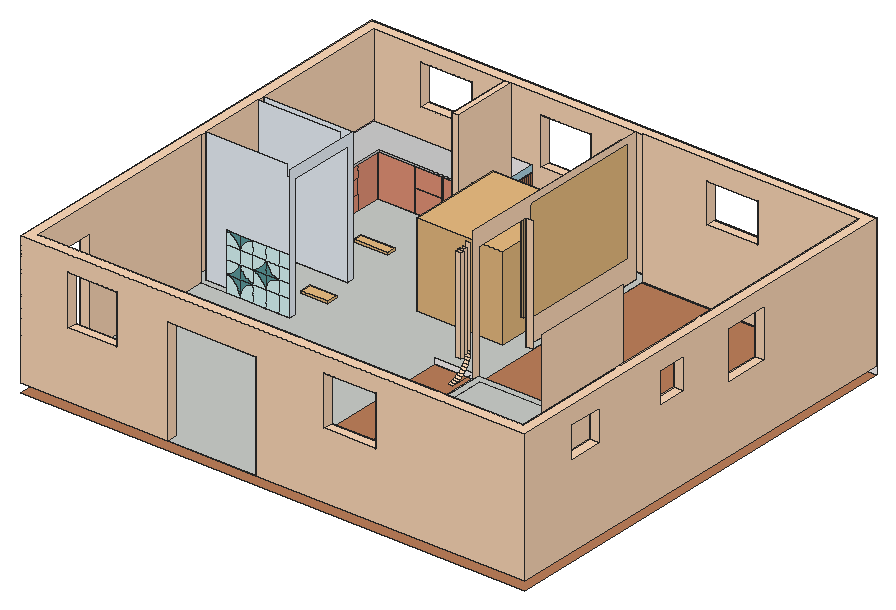
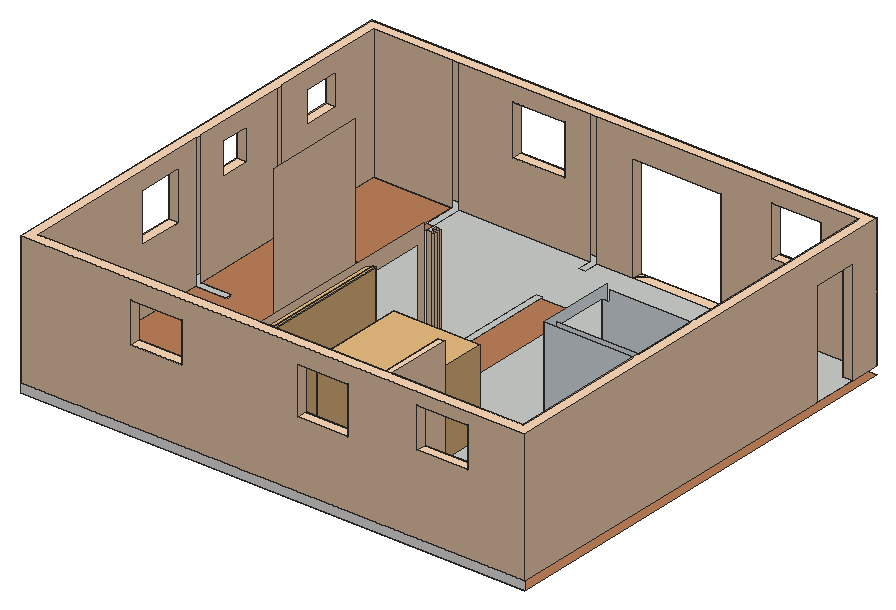
# SketchUp Ruby script. Lengths in inches.
U = 1.inch
M = Sketchup.active_model
def pt(a) = Geom::Point3d.new(a.map { |v| v * U })
def face(e, loops, mat)
  f = e.add_face(loops[0].map { |a| pt(a) })
  loops[1..].each { |l| e.add_face(l.map { |a| pt(a) }).erase! }
  f.material = f.back_material = mat if mat
  f
end
# faces: each face lists its corners as indices into pts; further lists are holes
def faces(e, pts, list, mat = nil) = list.each { |f| face(e, (f[0].is_a?(Array) ? f : [f]).map { |l| l.map { |i| pts[i] } }, mat) }
# xy, xz, yz: faces in a plane at the given z, y or x. An outline is a flat list of corners, or four numbers for a rectangle; further outlines are holes
def ring(l) = l.size == 4 ? [[l[0], l[1]], [l[2], l[1]], [l[2], l[3]], [l[0], l[3]]] : l.each_slice(2).to_a
def flat(e, list, mat, &to3) = list.each { |f| face(e, (f[0].is_a?(Array) ? f : [f]).map { |l| ring(l).map { |u, v| to3.(u, v) } }, mat) }
def xy(e, z, list, mat = nil) = flat(e, list, mat) { |x, y| [x, y, z] }
def xz(e, y, list, mat = nil) = flat(e, list, mat) { |x, z| [x, y, z] }
def yz(e, x, list, mat = nil) = flat(e, list, mat) { |y, z| [x, y, z] }
def lines(e, pts, list) = list.each { |a, b| e.add_line(pt(pts[a]), pt(pts[b])) }
# prism: a flat outline (further loops are holes) pulled along v
def prism(e, loops, v, mat = nil)
  f = face(e, loops, mat); d = Geom::Vector3d.new(v.map { |x| x * U })
  f.pushpull(f.normal.samedirection?(d) ? d.length : -d.length)
end
def box(e, o, s, mat = nil) = prism(e, [[o, [o[0] + s[0], o[1], o[2]], [o[0] + s[0], o[1] + s[1], o[2]], [o[0], o[1] + s[1], o[2]]]], [0, 0, s[2]], mat)
def at(x, y, z, deg = 0) = Geom::Transformation.translation(pt([x, y, z])) * Geom::Transformation.rotation(ORIGIN, Z_AXIS, deg.degrees)
def axes(o, x, y, z) = Geom::Transformation.new([*x, 0, *y, 0, *z, 0, *pt(o).to_a, 1])
def part(name) = M.definitions.add(name)
# library, detail: a bought-in or finely detailed component or shape, given as its bounding box
def library(name, o, s) = part(name).tap { |d| box(d.entities, o, s) }
def detail(e, o, s) = box(e.add_group.entities, o, s)
def put(e, d, t, mat = nil) = e.add_instance(d, t).tap { |i| i.material = mat if mat }
def group(e, t, mat = nil) = e.add_group.tap { |g| g.transformation = t; g.material = mat if mat }.entities
root = M.entities
M.materials.add("3D66_SU_1584934530570_001").color = [198, 166, 120]
M.materials.add("[0006_Pink]").color = [255, 192, 203]
M.materials.add("[0010_Snow]").color = [255, 250, 250]
M.materials.add("[0014_DarkSalmon]").color = [233, 150, 122]
M.materials.add("[0027_PeachPuff]").color = [255, 218, 185]
M.materials.add("[0081_CadetBlue]").color = [95, 158, 160]
M.materials.add("[0090_LightCyan]").color = [224, 255, 255]
M.materials.add("[0093_AliceBlue]").color = [240, 248, 255]
M.materials.add("[0095_LightBlue]").color = [173, 216, 230]
M.materials.add("[Basic Tile]").color = [203, 206, 202]
M.materials.add("[Carrera Marble]").color = [207, 207, 207]
M.materials.add("[Wood Veneer 02]").color = [190, 128, 91]
c1 = library("kitchen",[0.875,0,0],[30.86,8.22,2])
c2 = library("pooja",[0.875,0,0],[24.44,10.22,2])
c3 = library("Dining table set",[0,0,0],[63.25,59.01,43.49])
c4 = library("Dining ar",[0.98,0,0],[40.63,10.22,2])
c5 = part("\#79\#1")
prism(c5.entities,[[[1108.05,3703.68,-100.79],[497.03,3703.68,-100.79],[497.03,5166.16,-100.79],[1108.05,5166.16,-100.79]],[[1097.77,5155.88,-100.79],[507.31,5155.88,-100.79],[507.31,3713.96,-100.79],[1097.77,3713.96,-100.79]]],[0,0,14.57],"3D66_SU_1584934530570_001")
c6 = library("\#81",[507.31,3713.96,-116.94],[590.46,1441.92,47.04])
xy(root,-7.5625,[[109.5625,138.9375,571.5625,540.9375]],"[Wood Veneer 02]")
xy(root,0,[[[109.5625,138.9375,571.5625,540.9375],[490.5625,258.9375,490.5625,347.21,492.04,347.21,492.04,350.1875,490.5625,350.1875,490.5625,351.9375,364.5625,351.9375,364.5625,531.9375,562.5625,531.9375,562.5625,351.9375,534.83,351.9375,534.83,350.1875,533.35,350.1875,533.35,348.7,535.05,348.7,535.05,345.9375,562.5625,345.9375,562.5625,258.9375],[490.5625,147.9375,490.5625,177.19,483.52,177.19,483.52,240.51,490.5625,240.51,490.5625,252.9375,562.5625,252.9375,562.5625,147.9375],[323.75,211.625,358.5625,345.9375],[118.5625,405.9375,139.41,531.9375],[244.5625,486.17,263.2,531.9375]]],"[Basic Tile]")
xy(root,6.75,[[263.2,488.05,263.89,509.17],[263.89,488.05,264.76,489.21],[263.89,490.54,264.76,491.71],[263.89,493.04,264.76,494.2],[263.89,495.53,264.76,496.7],
  [263.89,498.03,264.76,499.19],[263.89,500.52,264.76,501.6875],[263.89,503.02,264.76,504.18],[263.89,505.51,264.76,506.68],[263.89,508.01,264.76,509.17],
  [263.2,509.67,263.89,530],[263.89,510.01,264.76,511.17],[263.89,512.36,264.76,513.53],[263.89,514.71,264.76,515.88],[263.89,517.07,264.76,518.23],
  [263.89,519.42,264.76,520.59],[263.89,521.77,264.76,522.9375],[263.89,524.125,264.76,525.29],[263.89,526.48,264.76,527.65],[263.89,528.83,264.76,530]],"[0010_Snow]")
xy(root,23.08,[[354.3125,330.97,359.375,333.97],[354.3125,336.47,357.4375,339.47]],"[0027_PeachPuff]")
xy(root,44.75,[[118.58,405.9375,118.58,533.96,238.5625,533.96,238.5625,500.54,148.4,500.54,148.4,405.9375]],"[0006_Pink]")
xy(root,46.25,[[118.58,405.9375,148.4,405.9375,148.4,500.54,238.5625,500.54,238.5625,533.96,118.58,533.96]],"[Carrera Marble]")
xy(root,121.1875,[[238.5625,471.5,244.5625,531.9375]],"[0027_PeachPuff]")
xz(root,330.97,[[354.3125,23.08,359.375,110.27]],"[0027_PeachPuff]")
xz(root,333.9375,[[154.5625,0,154.5625,15.41,142.5625,15.41,144.1875,14.8125,145.74,14.05,147.22,13.14,148.59,12.09,149.85,10.9,150.98,9.59,151.97,8.17,152.82,6.66,153.5,5.07,154.03,3.42,154.38,1.72],[154.5625,0,154.6875,1.74,155,3.46,155.49,5.13,156.16,6.74,157,8.27,158,9.7,159.14,11.02,160.42,12.2,161.82,13.25,163.32,14.14,164.91,14.86,166.5625,15.41,154.5625,15.41],[142.5625,15.41,154.5625,15.41,154.5625,27.41,154.01,26.06,153.37,24.75,152.625,23.49,151.8,22.29,150.88,21.15,149.89,20.08,148.82,19.09,147.68,18.17,146.48,17.35,145.22,16.61,143.91,15.96],[154.5625,15.41,166.5625,15.41,165.19,15.93,163.86,16.55,162.59,17.27,161.37,18.09,160.22,19,159.15,19.99,158.15,21.07,157.24,22.22,156.42,23.43,155.7,24.71,155.08,26.04,154.5625,27.41],[178.5625,15.41,178.5625,27.41,166.5625,27.41,167.94,26.91,169.28,26.3,170.5625,25.58,171.79,24.77,172.94,23.86,174.02,22.87,175.02,21.79,175.93,20.63,176.74,19.41,177.45,18.125,178.0625,16.79],
  [178.5625,15.41,178.7,16.96,179.04,18.48,179.57,19.95,180.27,21.34,181.15,22.625,182.18,23.79,183.34,24.82,184.63,25.7,186.02,26.4,187.49,26.93,189.01,27.27,190.5625,27.41,178.5625,27.41],[166.5625,27.41,178.5625,27.41,178.5625,39.41,178.01,38.06,177.37,36.75,176.625,35.49,175.8,34.29,174.88,33.15,173.89,32.08,172.82,31.09,171.68,30.17,170.48,29.35,169.22,28.61,167.91,27.96],[178.5625,27.41,190.5625,27.41,189.12,27.79,187.72,28.3125,186.375,28.96,185.1,29.74,183.9,30.64,182.79,31.64,181.79,32.75,180.9,33.94,180.12,35.22,179.47,36.5625,178.95,37.96,178.5625,39.41],[154.5625,39.41,154.5625,51.41,142.5625,51.41,143.91,50.85,145.22,50.21,146.48,49.46,147.68,48.63,148.8125,47.72,149.88,46.73,150.875,45.66,151.79,44.52,152.62,43.32,153.36,42.06,154.01,40.76],[154.5625,39.41,155.0625,40.79,155.67,42.125,156.39,43.41,157.2,44.63,158.11,45.79,159.1,46.87,160.18,47.86,161.34,48.77,162.5625,49.58,163.85,50.3,165.18,50.91,166.5625,51.41,154.5625,51.41]],"[0081_CadetBlue]")
xz(root,333.9375,[[142.5625,0,154.5625,0,154.38,1.72,154.03,3.42,153.5,5.07,152.82,6.66,151.97,8.17,150.98,9.59,149.85,10.9,148.59,12.09,147.22,13.14,145.74,14.05,144.1875,14.8125,142.5625,15.41],[154.5625,0,166.5625,0,166.5625,15.41,164.91,14.86,163.32,14.14,161.82,13.25,160.42,12.2,159.14,11.02,158,9.7,157,8.27,156.16,6.74,155.49,5.13,155,3.46,154.6875,1.74],[166.5625,0,178.5625,15.41],[178.5625,0,190.5625,15.41],[190.5625,0,200.19,15.41],
  [142.5625,15.41,143.91,15.96,145.22,16.61,146.48,17.35,147.68,18.17,148.82,19.09,149.89,20.08,150.88,21.15,151.8,22.29,152.625,23.49,153.37,24.75,154.01,26.06,154.5625,27.41,142.5625,27.41],[166.5625,15.41,166.5625,27.41,154.5625,27.41,155.08,26.04,155.7,24.71,156.42,23.43,157.24,22.22,158.15,21.07,159.15,19.99,160.22,19,161.37,18.09,162.59,17.27,163.86,16.55,165.19,15.93],[166.5625,15.41,178.5625,15.41,178.0625,16.79,177.45,18.125,176.74,19.41,175.93,20.63,175.02,21.79,174.02,22.87,172.94,23.86,171.79,24.77,170.5625,25.58,169.28,26.3,167.94,26.91,166.5625,27.41],[178.5625,15.41,190.5625,15.41,190.5625,27.41,189.01,27.27,187.49,26.93,186.02,26.4,184.63,25.7,183.34,24.82,182.18,23.79,181.15,22.625,180.27,21.34,179.57,19.95,179.04,18.48,178.7,16.96],[190.5625,15.41,200.19,27.41],
  [142.5625,27.41,154.5625,39.41],[154.5625,27.41,166.5625,39.41],[166.5625,27.41,167.91,27.96,169.22,28.61,170.48,29.35,171.68,30.17,172.82,31.09,173.89,32.08,174.88,33.15,175.8,34.29,176.625,35.49,177.37,36.75,178.01,38.06,178.5625,39.41,166.5625,39.41],[190.5625,27.41,190.5625,39.41,178.5625,39.41,178.95,37.96,179.47,36.5625,180.12,35.22,180.9,33.94,181.79,32.75,182.79,31.64,183.9,30.64,185.1,29.74,186.375,28.96,187.72,28.3125,189.12,27.79],[190.5625,27.41,200.19,39.41],
  [142.5625,39.41,154.5625,39.41,154.01,40.76,153.36,42.06,152.62,43.32,151.79,44.52,150.875,45.66,149.88,46.73,148.8125,47.72,147.68,48.63,146.48,49.46,145.22,50.21,143.91,50.85,142.5625,51.41],[154.5625,39.41,166.5625,39.41,166.5625,51.41,165.18,50.91,163.85,50.3,162.5625,49.58,161.34,48.77,160.18,47.86,159.1,46.87,158.11,45.79,157.2,44.63,156.39,43.41,155.67,42.125,155.0625,40.79],[166.5625,39.41,178.5625,51.41],[178.5625,39.41,190.5625,51.41],[190.5625,39.41,200.19,51.41]],"[0090_LightCyan]")
xz(root,333.97,[[354.3125,23.08,359.375,110.27]],"[0027_PeachPuff]")
xz(root,336.47,[[354.3125,23.08,357.4375,110.27]],"[0027_PeachPuff]")
xz(root,339.47,[[354.3125,23.08,357.4375,110.27]],"[0027_PeachPuff]")
xz(root,339.9375,[[118.5625,0,118.5625,121.1875,193.07,121.1875,193.07,111.25,200.19,111.25,200.19,0]],"[0093_AliceBlue]")
xz(root,342.58,[[354.3125,24.64,358.5625,113.35]],"[0027_PeachPuff]")
xz(root,345.9375,[[323.75,0,358.5625,4.8125]],"[0010_Snow]")
xz(root,399.9375,[[118.5625,0,200.19,0,200.19,111.25,193.07,111.25,193.07,121.1875,118.5625,121.1875]],"[0093_AliceBlue]")
xz(root,405.9375,[[118.58,44.75,148.4,46.25]],"[0006_Pink]")
xz(root,405.9375,[[118.5625,0,200.19,121.1875]],"[0093_AliceBlue]")
xz(root,406.625,[[358.5625,0,364.5625,105.53]],"[0027_PeachPuff]")
xz(root,471.5,[[238.5625,0,244.5625,121.1875]],"[0027_PeachPuff]")
xz(root,486.17,[[244.5625,0,263.2,60.5]],"[0010_Snow]")
xz(root,488.05,[[263.2,6.75,263.89,54.75]],"[0010_Snow]")
xz(root,488.05,[[263.89,6.75,264.76,54.75]],"[Wood Veneer 02]")
xz(root,489.21,[[263.89,6.75,264.76,54.75]],"[Wood Veneer 02]")
xz(root,490.54,[[263.89,6.75,264.76,54.75]],"[Wood Veneer 02]")
xz(root,491.71,[[263.89,6.75,264.76,54.75]],"[Wood Veneer 02]")
xz(root,493.04,[[263.89,6.75,264.76,54.75]],"[Wood Veneer 02]")
xz(root,494.2,[[263.89,6.75,264.76,54.75]],"[Wood Veneer 02]")
xz(root,495.53,[[263.89,6.75,264.76,54.75]],"[Wood Veneer 02]")
xz(root,496.7,[[263.89,6.75,264.76,54.75]],"[Wood Veneer 02]")
xz(root,498.03,[[263.89,6.75,264.76,54.75]],"[Wood Veneer 02]")
xz(root,499.19,[[263.89,6.75,264.76,54.75]],"[Wood Veneer 02]")
xz(root,500.52,[[263.89,6.75,264.76,54.75]],"[Wood Veneer 02]")
xz(root,500.54,[[148.4,44.75,238.5625,46.25]],"[Carrera Marble]")
xz(root,501.6875,[[263.89,6.75,264.76,54.75]],"[Wood Veneer 02]")
xz(root,503.02,[[263.89,6.75,264.76,54.75]],"[Wood Veneer 02]")
xz(root,504.18,[[263.89,6.75,264.76,54.75]],"[Wood Veneer 02]")
xz(root,505.51,[[263.89,6.75,264.76,54.75]],"[Wood Veneer 02]")
xz(root,506.68,[[263.89,6.75,264.76,54.75]],"[Wood Veneer 02]")
xz(root,508.01,[[263.89,6.75,264.76,54.75]],"[Wood Veneer 02]")
xz(root,509.17,[[263.2,6.75,263.89,54.75]],"[0095_LightBlue]")
xz(root,509.17,[[263.89,6.75,264.76,54.75]],"[Wood Veneer 02]")
xz(root,509.67,[[263.2,6.75,263.89,54.75]],"[0010_Snow]")
xz(root,510.01,[[263.89,6.75,264.76,54.75]],"[Wood Veneer 02]")
xz(root,511.17,[[263.89,6.75,264.76,54.75]],"[Wood Veneer 02]")
xz(root,512.36,[[263.89,6.75,264.76,54.75]],"[Wood Veneer 02]")
xz(root,513.53,[[263.89,6.75,264.76,54.75]],"[Wood Veneer 02]")
xz(root,514.71,[[263.89,6.75,264.76,54.75]],"[Wood Veneer 02]")
xz(root,515.88,[[263.89,6.75,264.76,54.75]],"[Wood Veneer 02]")
xz(root,517.07,[[263.89,6.75,264.76,54.75]],"[Wood Veneer 02]")
xz(root,518.23,[[263.89,6.75,264.76,54.75]],"[Wood Veneer 02]")
xz(root,519.42,[[263.89,6.75,264.76,54.75]],"[Wood Veneer 02]")
xz(root,520.59,[[263.89,6.75,264.76,54.75]],"[Wood Veneer 02]")
xz(root,521.77,[[263.89,6.75,264.76,54.75]],"[Wood Veneer 02]")
xz(root,522.9375,[[263.89,6.75,264.76,54.75]],"[Wood Veneer 02]")
xz(root,524.125,[[263.89,6.75,264.76,54.75]],"[Wood Veneer 02]")
xz(root,525.29,[[263.89,6.75,264.76,54.75]],"[Wood Veneer 02]")
xz(root,526.48,[[263.89,6.75,264.76,54.75]],"[Wood Veneer 02]")
xz(root,527.65,[[263.89,6.75,264.76,54.75]],"[Wood Veneer 02]")
xz(root,528.83,[[263.89,6.75,264.76,54.75]],"[Wood Veneer 02]")
xz(root,530,[[263.2,6.75,263.89,54.75]],"[0010_Snow]")
xz(root,530,[[263.89,6.75,264.76,54.75]],"[Wood Veneer 02]")
xz(root,531.9375,[[244.5625,0,263.2,60.5]],"[0010_Snow]")
xz(root,533.96,[[118.58,44.75,238.5625,46.25]],"[0006_Pink]")
xz(root,540.9375,[[109.5625,-7.5625,571.5625,0]],"[0010_Snow]")
yz(root,118.58,[[405.9375,44.75,533.96,46.25]],"[0006_Pink]")
yz(root,148.4,[[405.9375,44.75,500.54,46.25]],"[Carrera Marble]")
yz(root,200.19,[[333.9375,0,339.9375,0,339.9375,111.25,399.9375,111.25,399.9375,0,405.9375,0,405.9375,121.1875,333.9375,121.1875]],"[0093_AliceBlue]")
yz(root,238.5625,[[500.54,44.75,533.96,46.25]],"[0006_Pink]")
yz(root,238.5625,[[471.5,0,531.9375,121.1875]],"[0027_PeachPuff]")
yz(root,244.5625,[[486.17,0,531.9375,60.5]],"[0010_Snow]")
yz(root,244.5625,[[471.5,0,531.9375,121.1875]],"[0027_PeachPuff]")
yz(root,263.2,[[[486.17,0,531.9375,60.5],[488.05,6.75,509.17,54.75],[509.67,6.75,530,54.75]]],"[0095_LightBlue]")
yz(root,263.89,[[488.05,6.75,489.21,54.75],[490.54,6.75,491.71,54.75],[493.04,6.75,494.2,54.75],[495.53,6.75,496.7,54.75],[498.03,6.75,499.19,54.75],
  [500.52,6.75,501.6875,54.75],[503.02,6.75,504.18,54.75],[505.51,6.75,506.68,54.75],[508.01,6.75,509.17,54.75],[510.01,6.75,511.17,54.75],
  [512.36,6.75,513.53,54.75],[514.71,6.75,515.88,54.75],[517.07,6.75,518.23,54.75],[519.42,6.75,520.59,54.75],[521.77,6.75,522.9375,54.75],
  [524.125,6.75,525.29,54.75]],"[0010_Snow]")
yz(root,263.89,[[489.21,6.75,490.54,54.75],[491.71,6.75,493.04,54.75],[494.2,6.75,495.53,54.75],[496.7,6.75,498.03,54.75],[499.19,6.75,500.52,54.75],
  [501.6875,6.75,503.02,54.75],[504.18,6.75,505.51,54.75],[506.68,6.75,508.01,54.75],[509.67,6.75,510.01,54.75],[511.17,6.75,512.36,54.75],
  [513.53,6.75,514.71,54.75],[515.88,6.75,517.07,54.75],[518.23,6.75,519.42,54.75],[520.59,6.75,521.77,54.75],[522.9375,6.75,524.125,54.75],
  [525.29,6.75,526.48,54.75],[526.48,6.75,527.65,54.75],[527.65,6.75,528.83,54.75],[528.83,6.75,530,54.75]],"[0095_LightBlue]")
yz(root,264.76,[[488.05,6.75,489.21,54.75],[490.54,6.75,491.71,54.75],[493.04,6.75,494.2,54.75],[495.53,6.75,496.7,54.75],[498.03,6.75,499.19,54.75],
  [500.52,6.75,501.6875,54.75],[503.02,6.75,504.18,54.75],[505.51,6.75,506.68,54.75],[508.01,6.75,509.17,54.75],[510.01,6.75,511.17,54.75],
  [512.36,6.75,513.53,54.75],[514.71,6.75,515.88,54.75],[517.07,6.75,518.23,54.75],[519.42,6.75,520.59,54.75],[521.77,6.75,522.9375,54.75],
  [524.125,6.75,525.29,54.75],[526.48,6.75,527.65,54.75],[528.83,6.75,530,54.75]],"[Wood Veneer 02]")
yz(root,357.4375,[[336.47,23.08,339.47,110.27]],"[0027_PeachPuff]")
yz(root,358.5625,[[345.9375,0,345.9375,121.1875,531.9375,121.1875,531.9375,0,406.625,0,406.625,105.53,351.9375,105.53,351.9375,0]],"[0027_PeachPuff]")
yz(root,359.375,[[330.97,23.08,333.97,110.27]],"[0027_PeachPuff]")
p = [[354.3125,322.76,4.8125],[354.3125,325.34,4.98],[358.5625,325.34,4.98],[358.5625,322.76,4.8125],[354.3125,327.89,5.49],[358.5625,327.89,5.49],
  [354.3125,330.34,6.32],[358.5625,330.34,6.32],[354.3125,332.67,7.47],[358.5625,332.67,7.47],[354.3125,334.83,8.91],[358.5625,334.83,8.91],
  [354.3125,336.78,10.62],[358.5625,336.78,10.62],[354.3125,338.49,12.57],[358.5625,338.49,12.57],[354.3125,339.93,14.73],[358.5625,339.93,14.73],
  [354.3125,341.08,17.05],[358.5625,341.08,17.05],[354.3125,341.91,19.51],[358.5625,341.91,19.51],[354.3125,342.42,22.05],[358.5625,342.42,22.05],
  [354.3125,342.58,24.64],[358.5625,342.58,24.64],[358.5625,342.58,4.8125]]
faces(root,p,[[0,1,2,3],[1,4,5,2],[4,6,7,5],[6,8,9,7],[8,10,11,9],[10,12,13,11],[12,14,15,13],[14,16,17,15],
  [16,18,19,17],[18,20,21,19],[20,22,23,21],[22,24,25,23]],"[0027_PeachPuff]")
lines(root,p,[[3,26]])
g1 = group(root,at(118.5625,405.9375,0),"[0010_Snow]")
g2 = group(g1,at(0,0,0))
xy(g2,0,[[20.85,102.47,120,126]],"[0014_DarkSalmon]")
xy(g2,4.5,[[20.85,0,20.85,102.47,29.52,102.47,29.52,97.28,26.52,97.28,26.52,0],[29.52,97.28,120,102.47],[20.85,102.47,120,126]],"[0014_DarkSalmon]")
xy(g2,5,[[26.52,1,27.65,24.73],[26.52,25.1875,27.65,38.75],[26.52,39.25,27.65,73],[26.52,73.5,27.65,95.78],[28.02,95.97,61.46,97.28],
  [61.96,95.97,86.46,97.28],[86.96,95.97,118.5,97.28]],"[0014_DarkSalmon]")
xy(g2,17.75,[[26.52,39.25,27.65,73]],"[0014_DarkSalmon]")
xy(g2,18.25,[[26.52,39.25,27.65,73]],"[0014_DarkSalmon]")
xy(g2,25.68,[[61.96,95.97,86.46,97.28]],"[0014_DarkSalmon]")
xy(g2,26.18,[[61.96,95.97,86.46,97.28]],"[0014_DarkSalmon]")
xy(g2,31.75,[[26.52,39.25,27.65,73]],"[0014_DarkSalmon]")
xy(g2,32.25,[[26.52,39.25,27.65,73]],"[0014_DarkSalmon]")
xy(g2,44.25,[[26.52,1,27.65,24.73],[26.52,25.1875,27.65,38.75],[26.52,39.25,27.65,73],[26.52,73.5,27.65,95.78],[28.02,95.97,61.46,97.28],
  [61.96,95.97,86.46,97.28],[86.96,95.97,118.5,97.28]],"[0014_DarkSalmon]")
xy(g2,44.75,[[0,0,26.52,0,26.52,97.28,120,97.28,120,126,0,126]],"[0014_DarkSalmon]")
xz(g2,0,[[0,4.5,20.85,44.75],[20.85,4.5,26.52,44.75]],"[0014_DarkSalmon]")
xz(g2,1,[[26.52,5,27.65,44.25]],"[0014_DarkSalmon]")
xz(g2,24.73,[[26.52,5,27.65,44.25]],"[0014_DarkSalmon]")
xz(g2,25.1875,[[26.52,5,27.65,44.25]],"[0014_DarkSalmon]")
xz(g2,38.75,[[26.52,5,27.65,44.25]],"[0014_DarkSalmon]")
xz(g2,39.25,[[26.52,5,27.65,17.75],[26.52,18.25,27.65,31.75],[26.52,32.25,27.65,44.25]],"[0014_DarkSalmon]")
xz(g2,73,[[26.52,5,27.65,17.75],[26.52,18.25,27.65,31.75],[26.52,32.25,27.65,44.25]],"[0014_DarkSalmon]")
xz(g2,73.5,[[26.52,5,27.65,44.25]],"[0014_DarkSalmon]")
xz(g2,95.78,[[26.52,5,27.65,44.25]],"[0014_DarkSalmon]")
xz(g2,95.97,[[28.02,5,61.46,44.25],[61.96,5,86.46,25.68],[86.96,5,118.5,44.25],[61.96,26.18,86.46,44.25]],"[0014_DarkSalmon]")
xz(g2,97.28,[[[26.52,4.5,120,44.75],[28.02,5,61.46,44.25],[86.96,5,118.5,44.25],[61.96,5,86.46,44.25]],[61.96,25.68,86.46,26.18]],"[0014_DarkSalmon]")
xz(g2,102.47,[[20.85,0,120,4.5]],"[0014_DarkSalmon]")
xz(g2,126,[[20.85,0,120,4.5],[0,4.5,120,44.75]],"[0014_DarkSalmon]")
yz(g2,0,[[0,4.5,126,44.75]],"[0014_DarkSalmon]")
yz(g2,20.85,[[0,0,102.47,4.5]],"[0014_DarkSalmon]")
yz(g2,26.52,[[0,4.5,1,44.75],[1,4.5,24.73,5],[24.73,4.5,25.1875,44.75],[25.1875,4.5,38.75,5],[[38.75,4.5,97.28,44.75],[73.5,5,95.78,44.25],[39.25,18.25,73,31.75],[39.25,5,73,17.75],[39.25,32.25,73,44.25]],
  [1,44.25,24.73,44.75],[25.1875,44.25,38.75,44.75]],"[0014_DarkSalmon]")
yz(g2,27.65,[[1,5,24.73,44.25],[25.1875,5,38.75,44.25],[39.25,5,73,17.75],[73.5,5,95.78,44.25],[39.25,18.25,73,31.75],
  [39.25,32.25,73,44.25]],"[0014_DarkSalmon]")
yz(g2,28.02,[[95.97,5,97.28,44.25]],"[0014_DarkSalmon]")
yz(g2,61.46,[[95.97,5,97.28,44.25]],"[0014_DarkSalmon]")
yz(g2,61.96,[[95.97,5,97.28,25.68],[95.97,26.18,97.28,44.25]],"[0014_DarkSalmon]")
yz(g2,86.46,[[95.97,5,97.28,25.68],[95.97,26.18,97.28,44.25]],"[0014_DarkSalmon]")
yz(g2,86.96,[[95.97,5,97.28,44.25]],"[0014_DarkSalmon]")
yz(g2,118.5,[[95.97,5,97.28,44.25]],"[0014_DarkSalmon]")
yz(g2,120,[[102.47,0,126,4.5],[97.28,4.5,126,44.75]],"[0014_DarkSalmon]")
put(root,c1,at(165.74,449.02,0))
put(root,c2,at(183.17,367.12,0))
put(root,c3,axes([265.26,397.9375,0],[1.25,0,0],[0,1.484,0],[0,0,1.7625]),"[0006_Pink]")
put(root,c4,at(289.2,501.64,0))
g3 = group(root,at(109.5625,138.9375,0),"[0027_PeachPuff]")
xy(g3,0,[[135,0,215.99,9]])
xy(g3,60.59,[[43.83,0,88.47,9],[277.57,0,325.5625,9],[453,232.22,462,274.68]])
xy(g3,61.625,[[162.09,393,208.3,402]])
xy(g3,67.48,[[313.84,393,360.72,402]])
xy(g3,72.6875,[[52.38,393,98.79,402]])
xy(g3,76.09,[[453,52.35,462,85.45],[453,154.42,462,181.83]])
xy(g3,95.4375,[[0,27,9,68.4375]])
xy(g3,97.6875,[[135,0,215.99,9]])
xy(g3,103.875,[[313.84,393,360.72,402]])
xy(g3,104.9375,[[453,52.35,462,85.45],[453,154.42,462,181.83],[453,232.22,462,274.68],[162.09,393,208.3,402]])
xy(g3,106.41,[[43.83,0,88.47,9],[277.57,0,325.5625,9]])
xy(g3,109.625,[[52.38,393,98.79,402]])
xy(g3,121.1875,[[[0,0,462,402],[9,9,453,393]]])
xz(g3,0,[[[0,0,135,0,135,97.6875,215.99,97.6875,215.99,0,462,0,462,121.1875,0,121.1875],[277.57,60.59,325.5625,106.41],[43.83,60.59,88.47,106.41]]])
xz(g3,9,[[[9,0,9,121.1875,249,121.1875,249,0,215.99,0,215.99,97.6875,135,97.6875,135,0],[43.83,60.59,88.47,106.41]],[[255,0,375,121.1875],[277.57,60.59,325.5625,106.41]],[381,0,453,121.1875]])
xz(g3,27,[[0,0,9,95.4375]])
xz(g3,52.35,[[453,76.09,462,104.9375]])
xz(g3,68.4375,[[0,0,9,95.4375]])
xz(g3,85.45,[[453,76.09,462,104.9375]])
xz(g3,154.42,[[453,76.09,462,104.9375]])
xz(g3,181.83,[[453,76.09,462,104.9375]])
xz(g3,232.22,[[453,60.59,462,104.9375]])
xz(g3,274.68,[[453,60.59,462,104.9375]])
xz(g3,393,[[[9,0,129,121.1875],[52.38,72.6875,98.79,109.625]],[[135,0,249,121.1875],[162.09,61.625,208.3,104.9375]],[[255,0,453,121.1875],[313.84,67.48,360.72,103.875]]])
xz(g3,402,[[[0,0,462,121.1875],[162.09,61.625,208.3,104.9375],[52.38,72.6875,98.79,109.625],[313.84,67.48,360.72,103.875]]])
yz(g3,0,[[0,0,0,121.1875,402,121.1875,402,0,68.4375,0,68.4375,95.4375,27,95.4375,27,0]])
yz(g3,9,[[9,0,27,0,27,95.4375,68.4375,95.4375,68.4375,0,195,0,195,121.1875,9,121.1875],[201,0,261,121.1875],[267,0,393,121.1875]])
yz(g3,43.83,[[0,60.59,9,106.41]])
yz(g3,52.38,[[393,72.6875,402,109.625]])
yz(g3,88.47,[[0,60.59,9,106.41]])
yz(g3,98.79,[[393,72.6875,402,109.625]])
yz(g3,135,[[0,0,9,97.6875]])
yz(g3,162.09,[[393,61.625,402,104.9375]])
yz(g3,208.3,[[393,61.625,402,104.9375]])
yz(g3,215.99,[[0,0,9,97.6875]])
yz(g3,277.57,[[0,60.59,9,106.41]])
yz(g3,313.84,[[393,67.48,402,103.875]])
yz(g3,325.5625,[[0,60.59,9,106.41]])
yz(g3,360.72,[[393,67.48,402,103.875]])
yz(g3,381,[[120,0,213,121.1875]])
yz(g3,453,[[[9,0,114,121.1875],[52.35,76.09,85.45,104.9375]],[[120,0,207,121.1875],[154.42,76.09,181.83,104.9375]],[[213,0,393,121.1875],[232.22,60.59,274.68,104.9375]]])
yz(g3,462,[[[0,0,402,121.1875],[232.22,60.59,274.68,104.9375],[52.35,76.09,85.45,104.9375],[154.42,76.09,181.83,104.9375]]])
p = [[0,68.4375,0],[0,27,0],[135,332.5625,0],[129,332.5625,0],[425.27,213,0],[453,213,0],
  [375,107.26,0],[375,207,0],[453,207,0],[425.27,207,0],[381,213,0],[249,213,0],
  [255,393,0],[255,267.6875,0],[381,107.26,0],[249,207,0],[249,21.68,0],[249,9,0],
  [375,21,0],[375,9,0],[249,70.55,0],[255,70.55,0],[135,393,0],[9,201,0],
  [90.63,201,0],[90.63,267,0],[9,267,0],[453,120,0],[381,120,0],[249,267.6875,0],
  [255,207,0],[381,114,0],[381,21,0],[381,9,0],[90.63,195,0],[9,195,0],
  [129,393,0],[375,68.84,0],[90.63,261,0],[249,393,0],[255,9,0],[255,21.68,0],
  [381,68.84,0],[9,261,0],[453,114,0]]
lines(g3,p,[[0,1],[2,3],[4,5],[6,7],[8,9],[10,11],[12,13],[9,4],[14,6],[15,11],[16,17],[18,19],
  [20,21],[22,2],[23,24],[25,26],[27,28],[29,13],[21,30],[31,14],[32,33],[34,35],[3,36],[30,7],
  [18,37],[38,25],[29,39],[40,41],[42,32],[41,16],[43,38],[24,34],[37,42],[15,20],[31,44]])
put(root,c5,axes([367.77,316.67,-219.49],[0,0.18694,0],[0,0,0.06481],[0.15997,0,0]),"3D66_SU_1584934530570_001")
put(root,c6,axes([369.75,316.67,-219.49],[0,0.18694,0],[0,0,0.06481],[0.16002,0,0]),"3D66_SU_1584934530570_001")
